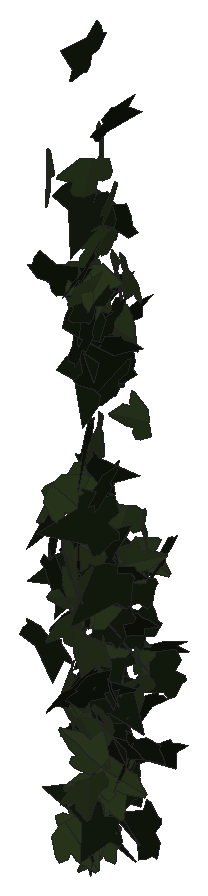
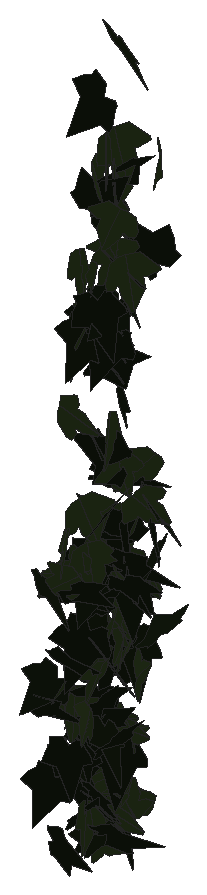
# SketchUp Ruby script. Lengths in inches.
U = 1.inch
M = Sketchup.active_model
def pt(a) = Geom::Point3d.new(a.map { |v| v * U })
def face(e, loops, mat)
  f = e.add_face(loops[0].map { |a| pt(a) })
  loops[1..].each { |l| e.add_face(l.map { |a| pt(a) }).erase! }
  f.material = f.back_material = mat if mat
  f
end
# faces: each face lists its corners as indices into pts; further lists are holes
def faces(e, pts, list, mat = nil) = list.each { |f| face(e, (f[0].is_a?(Array) ? f : [f]).map { |l| l.map { |i| pts[i] } }, mat) }
# xy, xz, yz: faces in a plane at the given z, y or x. An outline is a flat list of corners, or four numbers for a rectangle; further outlines are holes
def ring(l) = l.size == 4 ? [[l[0], l[1]], [l[2], l[1]], [l[2], l[3]], [l[0], l[3]]] : l.each_slice(2).to_a
def flat(e, list, mat, &to3) = list.each { |f| face(e, (f[0].is_a?(Array) ? f : [f]).map { |l| ring(l).map { |u, v| to3.(u, v) } }, mat) }
def xy(e, z, list, mat = nil) = flat(e, list, mat) { |x, y| [x, y, z] }
def xz(e, y, list, mat = nil) = flat(e, list, mat) { |x, z| [x, y, z] }
def yz(e, x, list, mat = nil) = flat(e, list, mat) { |y, z| [x, y, z] }
def lines(e, pts, list) = list.each { |a, b| e.add_line(pt(pts[a]), pt(pts[b])) }
# prism: a flat outline (further loops are holes) pulled along v
def prism(e, loops, v, mat = nil)
  f = face(e, loops, mat); d = Geom::Vector3d.new(v.map { |x| x * U })
  f.pushpull(f.normal.samedirection?(d) ? d.length : -d.length)
end
def box(e, o, s, mat = nil) = prism(e, [[o, [o[0] + s[0], o[1], o[2]], [o[0] + s[0], o[1] + s[1], o[2]], [o[0], o[1] + s[1], o[2]]]], [0, 0, s[2]], mat)
def at(x, y, z, deg = 0) = Geom::Transformation.translation(pt([x, y, z])) * Geom::Transformation.rotation(ORIGIN, Z_AXIS, deg.degrees)
def axes(o, x, y, z) = Geom::Transformation.new([*x, 0, *y, 0, *z, 0, *pt(o).to_a, 1])
def part(name) = M.definitions.add(name)
# library, detail: a bought-in or finely detailed component or shape, given as its bounding box
def library(name, o, s) = part(name).tap { |d| box(d.entities, o, s) }
def detail(e, o, s) = box(e.add_group.entities, o, s)
def put(e, d, t, mat = nil) = e.add_instance(d, t).tap { |i| i.material = mat if mat }
def group(e, t, mat = nil) = e.add_group.tap { |g| g.transformation = t; g.material = mat if mat }.entities
root = M.entities
M.materials.add("efeu1").color = [18, 25, 13]
M.materials.add("efeu2").color = [43, 57, 29]
c1 = part("ivyleaf_9")
p = [[1.54,2.16,1.25],[1.36,2.04,1.19],[-0.21,0.99,0.68],[-0.71,1.11,0.82],[-0.85,0.86,0.67],[-0.8,0.17,0.21],
  [-0.9,-0.01,0.1],[-0.67,-0.16,-0.02],[-0.08,-0.08,-0.05],[-0.03,-0.6,-0.4],[0.65,-0.88,-0.66],[0.83,-0.6,-0.49],
  [1.29,-0.42,-0.43],[1.8125,-0.07,-0.26],[1.21,0.44,0.15]]
faces(c1.entities,p,[[0,1,2,3,4,5,6,7,8,9,10,11,12,13,14]],"efeu1")
c2 = part("ivyleaf_10")
p = [[0,0.5,-0.03],[-0.0625,2.02,-0.43],[-0.19,2.01,-0.46],[-0.54,1.05,-0.29],[-0.52,0.625,-0.18],[-0.83,0.76,-0.28],
  [-1.16,0.64,-0.33],[-1.15,0.33,-0.24],[-0.77,-0.39,0.02],[-0.3,-0.51,0.16],[0.04,-0.48,0.23],[-0.02,2.01,-0.4375],
  [-0.06,2.01,-0.43],[0.04,-0.49,0.23],[0.67,-0.49,0.14],[1.38,0.36,-0.2],[1.375,0.51,-0.24],[0.81,0.65,-0.19],
  [0.62,0.59,-0.15],[0.6,1.09,-0.28],[0.5,1.23,-0.31]]
faces(c2.entities,p,[[0,1,2,3,4,5,6,7,8,9,10],[11,12,0,13,14,15,16,17,18,19,20]],"efeu2")
put(root,c1,axes([503.3,131.65,215.85],[0.01034,-0.79594,0.43319],[0.33885,-0.3984,-0.74009],[0.84045,0.17041,0.29306]))
put(root,c2,axes([505.84,131.12,210.26],[-0.28011,-0.85652,-0.09313],[0.04271,0.08158,-0.93061],[0.9291,-0.26198,0.0147]))
put(root,c2,axes([504.86,130.95,220.63],[-0.46983,0.82348,0.04425],[-0.01681,0.0399,-0.96856],[-0.89038,-0.43527,-0.00506]))
put(root,c1,axes([505.56,131.51,226.25],[-0.40053,0.07938,-0.77615],[0.74522,-0.29136,-0.38884],[-0.31881,-0.78078,0.0662]))
put(root,c1,axes([503.83,131.26,232.5625],[-0.03195,-0.1858,0.86569],[0.81935,-0.38626,-0.06162],[0.42083,0.73794,0.18571]))
put(root,c1,axes([505.35,130.71,214.71],[-0.0712,0.94192,0.04872],[-0.01444,0.04602,-0.98193],[-1.01843,-0.0665,0.01051]))
put(root,c1,axes([505.89,131.25,234.4375],[-0.63204,0.53033,-0.2769],[0.22767,-0.16375,-0.82112],[-0.59908,-0.62174,-0.01992]))
put(root,c2,axes([505.04,131.05,217.59],[-0.31069,-0.79702,-0.32479],[0.10812,0.29588,-0.88122],[0.91816,-0.30454,-0.00614]))
put(root,c1,axes([506.23,131.68,222.15],[-0.78189,-0.05192,0.56352],[-0.55806,-0.21792,-0.73974],[0.18483,-0.87763,0.15034]))
put(root,c2,axes([505.73,131.2,216.68],[-0.95091,-0.02652,0.30391],[-0.31519,-0.01672,-0.91607],[0.03287,-0.92754,0.00782]))
put(root,c2,axes([503.375,131.67,237.7],[-0.40455,0.6193,-0.48798],[0.08152,-0.48942,-0.73449],[-0.83516,-0.34776,0.16468]))
put(root,c1,axes([505.21,132.16,236.52],[-0.31426,-0.89178,0.1999],[-0.0093,-0.20826,-0.94368],[0.91386,-0.30879,0.05914]))
put(root,c2,axes([504.42,131.1,223.15],[0.27881,0.5531,0.64588],[0.30129,0.55499,-0.63466],[-0.84612,0.37988,-0.01317]))
put(root,c2,axes([504.875,131.43,218.36],[-0.32914,0.10261,0.82971],[-0.8675,0.00628,-0.31995],[-0.04593,-0.854,0.09734]))
put(root,c1,axes([505.63,130.93,230.32],[-0.03592,0.36685,0.88285],[-0.25503,0.81792,-0.37722],[-0.96565,-0.22966,0.06679]))
put(root,c1,axes([505.64,132.25,208.22],[-0.28403,-0.7347,0.40293],[0.08619,-0.44881,-0.75759],[0.83349,-0.20395,0.21565]))
put(root,c2,axes([505.11,132.08,218.96],[0.27693,-0.58183,0.5827],[0.2428,-0.51321,-0.66126],[0.83789,0.34101,-0.00098]))
put(root,c2,axes([505.79,132.06,234.87],[-0.0278,-0.8184,0.50388],[-0.02804,-0.50318,-0.81882],[0.96067,-0.03837,-0.00932]))
put(root,c2,axes([504.83,131.3,207.64],[0.45307,0.66065,0.50455],[0.28224,0.40875,-0.81389],[-0.83902,0.49425,-0.00133]))
put(root,c1,axes([503.9,131.74,222.03],[-0.74552,0.38847,-0.22037],[0.19321,-0.11412,-0.8237],[-0.4371,-0.71301,0.01177]))
put(root,c1,axes([503.51,131.67,219.32],[0.61617,-0.53941,-0.24094],[-0.18443,0.1566,-0.81655],[0.6066,0.59553,-0.00352]))
put(root,c2,axes([505.29,131.9375,237.95],[-0.39996,-0.86683,0.17718],[-0.0243,-0.18361,-0.95313],[0.88442,-0.39705,0.05394]))
put(root,c2,axes([503.9375,132.33,214],[-0.13739,0.17351,-0.79159],[0.07409,-0.76572,-0.19346],[-0.83986,-0.09594,0.11243]))
put(root,c1,axes([505.03,131.43,217.85],[0.06909,0.90864,-0.04104],[-0.06491,-0.03525,-0.94544],[-0.98011,0.06639,0.05972]))
put(root,c2,axes([505.32,131.84,233.04],[0.69028,0.52375,0.12763],[0.11081,0.06839,-0.85929],[-0.5703,0.64722,-0.01249]))
put(root,c1,axes([506.19,131.92,223.83],[-0.64836,0.53803,-0.06293],[0.0442,-0.04499,-0.83837],[-0.58306,-0.6017,0.00642]))
put(root,c1,axes([505.23,131.35,214.26],[0.54782,0.4124,0.59888],[0.48639,0.35888,-0.67987],[-0.59041,0.67831,-0.00441]))
put(root,c1,axes([506.05,132.5,219.36],[-0.74036,-0.54519,0.12969],[-0.11477,-0.06281,-0.91927],[0.54852,-0.749,-0.01731]))
put(root,c1,axes([505.64,131.68,231.91],[-0.22365,0.47135,0.69076],[-0.56976,0.44448,-0.49911],[-0.67012,-0.53523,0.19383]))
put(root,c1,axes([505.87,132.35,228.35],[0.47287,0.14124,0.76361],[-0.75889,-0.21305,0.47841],[0.27597,-0.8279,0.00716]))
put(root,c2,axes([505.4,131.84,232.63],[-0.45613,-0.61387,-0.39301],[0.22559,0.31498,-0.7749],[0.74513,-0.47113,-0.00598]))
put(root,c2,axes([505.21,132.3125,215.9],[0.7758,-0.29699,0.30283],[0.28438,-0.12511,-0.80827],[0.34771,0.76494,-0.01462]))
put(root,c2,axes([505.15,132.24,210.75],[0.46332,0.17901,0.70527],[-0.68773,-0.2338,0.48313],[0.3175,-0.76763,0.01732]))
put(root,c1,axes([505.05,131.92,218.02],[-0.28911,0.02698,-0.83581],[-0.86843,-0.01347,0.27808],[-0.00461,0.84697,0.03104]))
put(root,c1,axes([504.67,132.62,230.64],[0.13686,-0.9303,0.09037],[0.01436,-0.08923,-0.94032],[0.93457,0.13761,0.00122]))
put(root,c1,axes([503.53,131.67,220.07],[0.16376,-0.08688,0.91743],[-0.04693,0.89316,0.09925],[-0.95618,-0.05872,0.15226]))
put(root,c2,axes([505.14,131.82,220.56],[-0.32387,-0.35988,-0.72143],[0.54122,0.48157,-0.48514],[0.64762,-0.58242,0.04465]))
put(root,c1,axes([504.93,132.0625,219.92],[-0.16421,-0.08354,0.83999],[0.87694,-0.01686,0.15715],[0.0013,0.82169,0.08863]))
put(root,c2,axes([504.41,132.15,216],[-0.59742,0.64494,-0.05186],[0.03514,-0.03779,-0.88366],[-0.69773,-0.55412,-0.0001]))
put(root,c1,axes([505.03,131.98,207.12],[0.14328,0.04771,-0.83737],[-0.86841,0.0719,-0.13335],[0.06841,0.81284,0.06095]))
put(root,c2,axes([505.36,132.03,217.39],[0.46038,0.67891,-0.23664],[0.13848,0.18815,0.83367],[0.76081,-0.44507,-0.00854]))
put(root,c1,axes([504.84,131.8,219.81],[0.00146,-0.12918,0.89088],[0.09161,0.85252,0.13357],[-0.93111,0.08367,0.01454]))
put(root,c2,axes([503.625,132.59,222.24],[0.44842,0.43292,-0.56674],[-0.48471,-0.31844,-0.61873],[-0.57449,0.60659,0.07966]))
put(root,c2,axes([504.3,132.53,232.68],[-0.4408,-0.83269,0.12018],[0.00893,-0.14031,-0.93934],[0.84127,-0.43482,0.07295]))
put(root,c1,axes([506.45,132.15,228.54],[-0.51847,0.54936,0.34787],[-0.26777,0.22706,-0.75792],[-0.64094,-0.53925,0.03525]))
put(root,c2,axes([504.63,132.28,207.46],[0.48657,0.74159,0.05959],[-0.06074,-0.03137,0.88633],[0.7415,-0.4892,0.0335]))
put(root,c2,axes([505.8,132.625,236.57],[0.41599,-0.76517,0.14449],[0.08464,-0.11607,-0.89072],[0.83562,0.39268,0.01828]))
put(root,c1,axes([504.45,132.71,219.16],[-0.76501,-0.05139,0.42322],[-0.43809,-0.03264,-0.73861],[0.06568,-0.81626,0.00289]))
put(root,c2,axes([504.55,132.65,223.46],[0.45136,0.65123,-0.22984],[-0.11177,-0.1961,-0.80453],[-0.73426,0.43017,-0.01882]))
put(root,c2,axes([505.24,132.17,236.6875],[0.22313,-0.50381,-0.70012],[-0.28482,0.61941,-0.56627],[0.86228,0.33497,-0.00588]))
put(root,c1,axes([504.82,132.99,228.47],[-0.4315,-0.81627,-0.11491],[0.03407,0.11193,-0.92305],[0.82362,-0.43229,-0.02201]))
put(root,c1,axes([505.73,132.23,229.94],[0.67889,0.50916,-0.08703],[-0.07077,-0.05205,-0.8413],[-0.55276,0.63201,0.00082]))
put(root,c1,axes([504.92,132.31,242.83],[-0.47958,0.63673,0.41511],[-0.2755,0.30838,-0.80676],[-0.76342,-0.51128,0.03037]))
put(root,c2,axes([504.52,132.64,211.77],[-0.83736,0.14353,-0.36263],[0.36905,-0.06961,-0.82003],[-0.17217,-0.84728,0.00594]))
put(root,c1,axes([504.66,132.63,223.72],[0.58108,0.17393,-0.59492],[0.52458,0.32161,0.57681],[0.37655,-0.71644,0.1145]))
put(root,c1,axes([505.34,132.47,214.65],[0.58123,0.02261,-0.63364],[-0.65846,0.02209,-0.55924],[0.00173,0.81262,0.03283]))
put(root,c2,axes([504.95,133.19,206.52],[0.20999,0.46249,-0.59623],[-0.31028,-0.49835,-0.51945],[-0.73251,0.34368,0.04911]))
put(root,c1,axes([505.86,132.84,235],[0.2789,-0.21784,0.81894],[-0.69508,0.4545,0.35027],[-0.54356,-0.69296,-0.02771]))
put(root,c1,axes([505.21,133.04,215.42],[-0.2421,-0.68456,-0.34417],[0.12467,0.31037,-0.74904],[0.81166,-0.25186,0.0124]))
put(root,c1,axes([503.84,133.1875,218.7],[-0.7425,-0.37106,-0.13825],[0.12716,0.06173,-0.81249],[0.40625,-0.69751,0.00163]))
put(root,c2,axes([504.6,132.89,207.3125],[0.33605,0.79565,-0.08509],[-0.01761,-0.08146,-0.88837],[-0.86365,0.31126,-0.015]))
put(root,c2,axes([505.1875,132.86,211.84],[-0.26226,0.07718,-0.81459],[-0.81487,0.21044,0.26484],[0.2419,0.79258,0.009]))
put(root,c2,axes([505.1875,132.63,215.04],[0.33058,0.64625,0.44048],[0.19683,0.38232,-0.74368],[-0.81094,0.35624,-0.00094]))
put(root,c1,axes([504.72,132.71,207.61],[0.92858,-0.0357,-0.06406],[-0.06468,0.04095,-0.89407],[0.04158,0.86103,0.03986]))
put(root,c2,axes([504.24,132.85,211.63],[0.27755,-0.03112,0.84987],[-0.87756,0.08689,0.2692],[-0.0996,-0.85222,-0.00359]))
put(root,c2,axes([504.92,132.79,225.4],[0.28261,-0.75864,-0.44209],[0.01518,0.46857,-0.79438],[0.87792,0.23611,0.15605]))
put(root,c1,axes([505.72,133.3125,216.64],[-0.35202,-0.69961,-0.06175],[0.00765,-0.06873,0.80185],[-0.75826,0.3241,0.03675]))
put(root,c2,axes([504.75,133,216.42],[-0.27425,0.73226,-0.09205],[0.0468,-0.07863,-0.80589],[-0.79522,-0.25716,-0.01569]))
put(root,c1,axes([505.73,132.78,219.22],[0.40958,0.64348,-0.25359],[-0.19293,-0.17681,-0.7742],[-0.7177,0.41475,0.0634]))
put(root,c1,axes([505.62,132.9,230.6],[-0.57842,0.64086,0.10335],[-0.06643,0.07811,-0.86859],[-0.69725,-0.53909,-0.00298]))
put(root,c2,axes([505.05,133.3,208.68],[0.59622,0.28207,-0.56481],[-0.54159,-0.21071,-0.64396],[-0.37883,0.74519,0.03171]))
put(root,c1,axes([505.65,132.43,239.92],[0.26976,0.62253,0.5844],[0.23809,0.51696,-0.69753],[-0.87387,0.33302,-0.00965]))
put(root,c2,axes([505.77,133.53,221.53],[-0.36978,-0.75062,0.3394],[0.00531,-0.37419,-0.82178],[0.82377,-0.33453,0.15765]))
put(root,c1,axes([505.36,133.03,211.18],[0.69659,0.36237,-0.30268],[-0.26427,-0.15848,-0.76921],[-0.42676,0.68964,-0.01772]))
put(root,c1,axes([504.38,133.55,221.93],[0.35788,-0.8283,-0.0312],[-0.00457,0.03201,-0.90227],[0.82888,0.3578,0.00849]))
put(root,c1,axes([505.11,133.35,211.98],[-0.73593,-0.31688,-0.21485],[-0.20233,-0.08706,0.78156],[-0.35491,0.7067,-0.00006]))
put(root,c2,axes([504.72,133.25,238.44],[0.5113,-0.63259,-0.30487],[0.00499,0.35717,-0.79384],[0.75297,0.4272,0.21228]))
put(root,c2,axes([504.21,133.25,235.38],[0.76807,0.25616,0.33317],[0.24536,0.28786,-0.76391],[-0.36883,0.72494,0.18561]))
put(root,c2,axes([506.07,133.31,229.96],[0.02182,0.07895,0.86378],[-0.89827,0.06707,0.01441],[-0.07067,-0.82809,0.08353]))
put(root,c1,axes([504.9,133.84,212.01],[0.26907,-0.68647,0.21641],[0.09381,-0.18978,-0.7593],[0.769,0.26335,0.01691]))
put(root,c2,axes([505.39,133.6,219.57],[-0.39913,-0.80342,0.07175],[-0.00719,-0.07651,-0.89668],[0.80659,-0.39825,0.02751]))
put(root,c1,axes([504.61,132.84,230.9],[0.29503,0.57558,0.54458],[0.06968,0.5363,-0.64808],[-0.83748,0.24739,0.13792]))
put(root,c1,axes([504.05,133.29,211.11],[0.55969,0.54688,-0.41967],[-0.32169,-0.2709,-0.78204],[-0.60969,0.64497,0.02737]))
put(root,c2,axes([504.4,133.91,208.52],[-0.08745,-0.76898,0.3322],[-0.03047,-0.33086,-0.77391],[0.83711,-0.09237,0.00654]))
put(root,c1,axes([505.65,132.96,218.21],[0.18933,0.80387,0.32765],[-0.04323,0.34367,-0.81819],[-0.86701,0.15841,0.11234]))
put(root,c2,axes([506.11,133.37,232.72],[-0.67072,0.33631,0.46479],[-0.46327,0.14216,-0.73119],[-0.38764,-0.7518,0.06965]))
put(root,c1,axes([504.82,133.68,216.01],[0.71642,-0.35127,0.15343],[0.14241,-0.06623,-0.78064],[0.38604,0.67632,0.00325]))
put(root,c1,axes([505.02,133.54,213.38],[-0.00031,-0.46627,-0.64048],[0.12082,0.60932,-0.47985],[0.82545,-0.08936,0.07]))
put(root,c2,axes([505.12,133.32,209.58],[0.30634,0.33047,0.71865],[0.44571,0.55483,-0.45213],[-0.6969,0.50011,0.02673]))
put(root,c1,axes([504.83,133.88,215.64],[-0.816,0.31104,-0.04551],[0.04908,0.00102,-0.87307],[-0.31049,-0.81727,-0.0184]))
put(root,c2,axes([504.27,133.98,208.41],[-0.25134,0.06871,0.84724],[-0.79359,-0.33552,-0.20822],[0.30456,-0.81757,0.15666]))
put(root,c1,axes([503.58,134.47,211.97],[-0.25524,-0.74024,0.3473],[-0.03759,-0.35282,-0.77963],[0.8168,-0.24755,0.07264]))
put(root,c1,axes([504.26,133.51,230.04],[0.64475,0.50744,-0.15297],[-0.14435,-0.06965,-0.81413],[-0.55203,0.61089,0.03423]))
put(root,c2,axes([505.07,133.77,232.58],[-0.55481,0.63153,0.02117],[-0.05001,-0.01146,-0.84546],[-0.68058,-0.51399,0.04486]))
put(root,c2,axes([506.33,133.89,225.9],[-0.14202,0.02392,0.82217],[-0.8463,-0.11261,-0.13202],[0.11582,-0.79346,0.04353]))
put(root,c1,axes([504.29,134.375,213.54],[-0.16381,-0.8486,0.05328],[-0.01742,-0.05089,-0.86423],[0.85009,-0.16456,-0.00745]))
put(root,c1,axes([505.61,133.37,209.6],[0.06561,0.23232,0.81148],[-0.07862,0.78085,-0.2359],[-0.87572,-0.0527,0.08198]))
put(root,c1,axes([504.08,134.28,207.67],[0.55995,-0.59977,0.31881],[0.28112,-0.17149,-0.81638],[0.61833,0.62111,0.08245]))
put(root,c1,axes([504.65,133.95,231.55],[0.02207,0.73917,-0.34993],[-0.04139,-0.33533,-0.76854],[-0.87614,0.03446,0.02749]))
put(root,c1,axes([505.77,134.51,218.21],[-0.68006,-0.39105,0.17578],[-0.15502,-0.08926,-0.77088],[0.43319,-0.64584,0.0001]))
put(root,c1,axes([503.98,134.21,207.33],[-0.47398,0.27178,0.69057],[-0.72205,0.02042,-0.50362],[-0.17145,-0.83734,0.21186]))
put(root,c1,axes([505.49,134.2,208.77],[-0.69264,0.25574,0.31231],[-0.31337,0.08239,-0.71745],[-0.28855,-0.70335,0.02951]))
put(root,c1,axes([504.33,133.88,212.08],[-0.33645,0.78651,0.05578],[-0.01293,0.05513,-0.85539],[-0.78838,-0.33656,-0.00978]))
put(root,c1,axes([504.7,134.77,208.53],[-0.22621,-0.78199,0.22793],[-0.05127,-0.22242,-0.81396],[0.81291,-0.23163,0.01209]))
put(root,c2,axes([505.55,134.3,213.25],[-0.3792,-0.7726,-0.13833],[0.03951,0.13464,-0.86032],[0.78389,-0.38053,-0.02355]))
put(root,c2,axes([503.09,134.55,216.6875],[-0.46925,0.51219,-0.37908],[0.18396,-0.33059,-0.69429],[-0.65354,-0.46081,0.07674]))
put(root,c1,axes([504.71,134.65,209.55],[-0.8494,0.01908,-0.06607],[0.06626,0.00778,-0.84957],[-0.01841,-0.85193,-0.00924]))
put(root,c1,axes([505.14,134.9,218.58],[-0.60862,-0.43031,0.20762],[-0.16196,-0.13248,-0.73727],[0.48604,-0.58299,0.01429]))
put(root,c2,axes([505.37,134.11,229.67],[-0.40218,0.55717,0.46384],[-0.26014,0.37543,-0.69693],[-0.72556,-0.44344,-0.00723]))
put(root,c1,axes([505.65,134.37,210.76],[0.38727,0.46714,-0.60312],[-0.46493,-0.39172,-0.60194],[-0.60482,0.60023,0.07654]))
put(root,c2,axes([505.57,134.01,218.9375],[-0.00704,-0.12677,0.78975],[0.2374,0.72748,0.12827],[-0.79686,0.21785,0.03124]))
put(root,c1,axes([505.03,134.11,216.32],[0.65993,0.55067,-0.1857],[-0.20628,-0.04073,-0.85383],[-0.5433,0.68435,0.09861]))
put(root,c2,axes([505.86,134.54,220.57],[-0.46909,0.53723,0.355],[-0.27928,0.22867,-0.71649],[-0.62814,-0.50287,0.05345]))
put(root,c1,axes([505.09,134.26,230.05],[0.18396,0.71052,0.33405],[0.05827,0.31725,-0.7596],[-0.84011,0.17759,0.02047]))
put(root,c1,axes([506.18,134.79,206.63],[-0.38519,0.01188,-0.75127],[-0.73277,-0.19259,0.37266],[-0.16612,0.822,0.09817]))
put(root,c2,axes([504.52,134.82,208.6],[0.04135,-0.78365,-0.3134],[0.02271,0.31469,-0.7839],[0.84369,0.02994,0.03646]))
put(root,c2,axes([503.87,134.82,215.45],[-0.07797,0.71902,0.21737],[-0.00103,0.20989,-0.75128],[-0.80869,-0.06959,-0.02]))
put(root,c2,axes([505.29,135.09,214.31],[-0.1074,0.70892,-0.06379],[0.00155,-0.06173,-0.74446],[-0.7685,-0.0992,0.00741]))
put(root,c2,axes([505.27,134.93,219.0625],[0.3461,0.23991,0.64499],[0.4788,0.43603,-0.41367],[-0.53527,0.54516,0.04702]))
put(root,c1,axes([505.37,135.19,215.23],[-0.18629,0.29742,0.65727],[-0.62359,0.30559,-0.31346],[-0.42448,-0.57946,0.17204]))
put(root,c1,axes([506.23,135.46,218.95],[-0.48893,0.58549,0.02187],[-0.01164,0.01824,-0.7697],[-0.63263,-0.45283,-0.00274]))
put(root,c1,axes([506.22,136.01,213.47],[-0.69176,-0.1175,0.29909],[-0.29496,-0.10112,-0.67558],[0.15992,-0.6948,0.04774]))
put(root,c2,axes([504.2,135.2,213.27],[0.12449,0.2938,0.67465],[-0.47076,0.54878,-0.17794],[-0.60821,-0.36462,0.27582]))
put(root,c1,axes([504.875,135.55,211.72],[0.10818,0.68776,-0.14491],[-0.02349,-0.13764,-0.72282],[-0.75751,0.10249,0.00172]))
put(root,c1,axes([505.77,135.42,209.93],[0.4206,0.58885,0.04114],[0.02102,0.03455,-0.73422],[-0.63705,0.38992,0.00293]))
put(root,c1,axes([505.65,135.49,214.61],[0.57382,0.43523,0.1979],[0.02162,0.26473,-0.68785],[-0.51256,0.49842,0.19254]))
